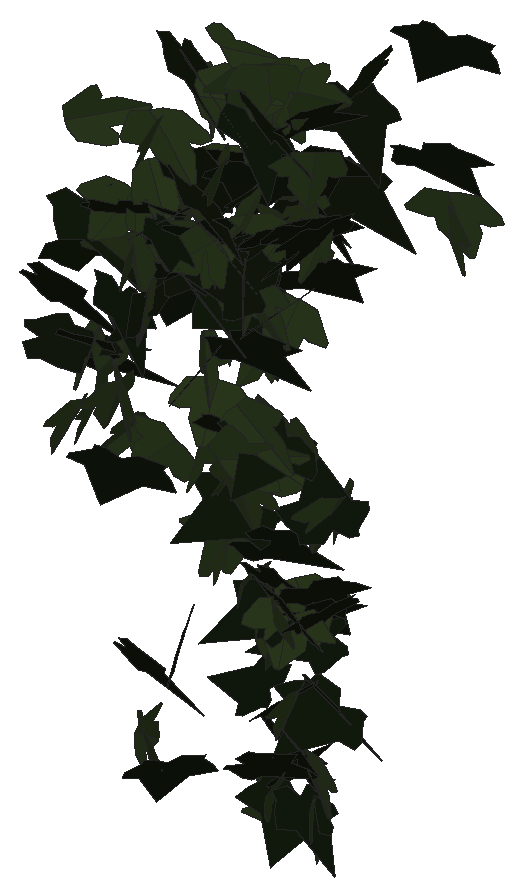
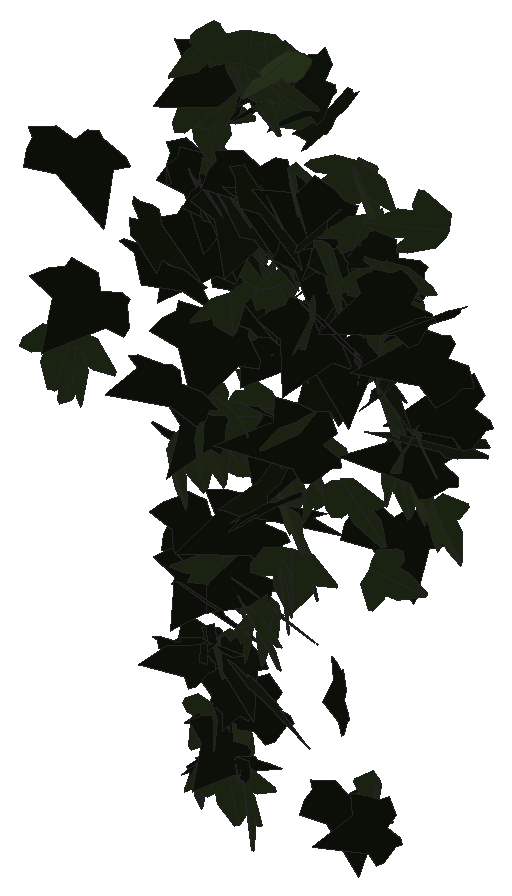
# SketchUp Ruby script. Lengths in inches.
U = 1.inch
M = Sketchup.active_model
def pt(a) = Geom::Point3d.new(a.map { |v| v * U })
def face(e, loops, mat)
  f = e.add_face(loops[0].map { |a| pt(a) })
  loops[1..].each { |l| e.add_face(l.map { |a| pt(a) }).erase! }
  f.material = f.back_material = mat if mat
  f
end
# faces: each face lists its corners as indices into pts; further lists are holes
def faces(e, pts, list, mat = nil) = list.each { |f| face(e, (f[0].is_a?(Array) ? f : [f]).map { |l| l.map { |i| pts[i] } }, mat) }
# xy, xz, yz: faces in a plane at the given z, y or x. An outline is a flat list of corners, or four numbers for a rectangle; further outlines are holes
def ring(l) = l.size == 4 ? [[l[0], l[1]], [l[2], l[1]], [l[2], l[3]], [l[0], l[3]]] : l.each_slice(2).to_a
def flat(e, list, mat, &to3) = list.each { |f| face(e, (f[0].is_a?(Array) ? f : [f]).map { |l| ring(l).map { |u, v| to3.(u, v) } }, mat) }
def xy(e, z, list, mat = nil) = flat(e, list, mat) { |x, y| [x, y, z] }
def xz(e, y, list, mat = nil) = flat(e, list, mat) { |x, z| [x, y, z] }
def yz(e, x, list, mat = nil) = flat(e, list, mat) { |y, z| [x, y, z] }
def lines(e, pts, list) = list.each { |a, b| e.add_line(pt(pts[a]), pt(pts[b])) }
# prism: a flat outline (further loops are holes) pulled along v
def prism(e, loops, v, mat = nil)
  f = face(e, loops, mat); d = Geom::Vector3d.new(v.map { |x| x * U })
  f.pushpull(f.normal.samedirection?(d) ? d.length : -d.length)
end
def box(e, o, s, mat = nil) = prism(e, [[o, [o[0] + s[0], o[1], o[2]], [o[0] + s[0], o[1] + s[1], o[2]], [o[0], o[1] + s[1], o[2]]]], [0, 0, s[2]], mat)
def at(x, y, z, deg = 0) = Geom::Transformation.translation(pt([x, y, z])) * Geom::Transformation.rotation(ORIGIN, Z_AXIS, deg.degrees)
def axes(o, x, y, z) = Geom::Transformation.new([*x, 0, *y, 0, *z, 0, *pt(o).to_a, 1])
def part(name) = M.definitions.add(name)
# library, detail: a bought-in or finely detailed component or shape, given as its bounding box
def library(name, o, s) = part(name).tap { |d| box(d.entities, o, s) }
def detail(e, o, s) = box(e.add_group.entities, o, s)
def put(e, d, t, mat = nil) = e.add_instance(d, t).tap { |i| i.material = mat if mat }
def group(e, t, mat = nil) = e.add_group.tap { |g| g.transformation = t; g.material = mat if mat }.entities
root = M.entities
M.materials.add("1026 AP 7946 SUNNY SIDE UP").color = [254, 231, 186]
M.materials.add("efeu1").color = [18, 25, 13]
M.materials.add("efeu2").color = [43, 57, 29]
c1 = part("ivyleaf_9")
p = [[1.54,2.16,1.25],[1.36,2.04,1.19],[-0.21,0.99,0.68],[-0.71,1.11,0.82],[-0.85,0.86,0.67],[-0.8,0.17,0.21],
  [-0.9,-0.01,0.1],[-0.67,-0.16,-0.02],[-0.08,-0.08,-0.05],[-0.03,-0.6,-0.4],[0.65,-0.88,-0.66],[0.83,-0.6,-0.49],
  [1.29,-0.42,-0.43],[1.8125,-0.07,-0.26],[1.21,0.44,0.15]]
faces(c1.entities,p,[[0,1,2,3,4,5,6,7,8,9,10,11,12,13,14]],"efeu1")
c2 = part("ivyleaf_10")
p = [[0,0.5,-0.03],[-0.0625,2.02,-0.43],[-0.19,2.01,-0.46],[-0.54,1.05,-0.29],[-0.52,0.625,-0.18],[-0.83,0.76,-0.28],
  [-1.16,0.64,-0.33],[-1.15,0.33,-0.24],[-0.77,-0.39,0.02],[-0.3,-0.51,0.16],[0.04,-0.48,0.23],[-0.02,2.01,-0.4375],
  [-0.06,2.01,-0.43],[0.04,-0.49,0.23],[0.67,-0.49,0.14],[1.38,0.36,-0.2],[1.375,0.51,-0.24],[0.81,0.65,-0.19],
  [0.62,0.59,-0.15],[0.6,1.09,-0.28],[0.5,1.23,-0.31]]
faces(c2.entities,p,[[0,1,2,3,4,5,6,7,8,9,10],[11,12,0,13,14,15,16,17,18,19,20]],"efeu2")
put(root,c1,axes([142.16,212.56,287.88],[0.31672,-0.17913,-0.21468],[-0.14461,0.19825,-0.26729],[0.40589,0.21041,0.07229]),"1026 AP 7946 SUNNY SIDE UP")
put(root,c1,axes([143.47,212.86,289.68],[-0.00222,-0.34743,0.04563],[0.00185,-0.04627,-0.35819],[0.55112,-0.00124,0.00138]),"1026 AP 7946 SUNNY SIDE UP")
put(root,c2,axes([140.59,212.77,284.56],[0.03264,-0.32635,0.0778],[0.00053,-0.0775,-0.33731],[0.52738,0.02028,-0.00447]),"1026 AP 7946 SUNNY SIDE UP")
put(root,c1,axes([142.63,212.65,290.1875],[0.46687,-0.18789,-0.08433],[-0.13261,0.01726,-0.36058],[0.29298,0.30723,-0.02883]),"1026 AP 7946 SUNNY SIDE UP")
put(root,c2,axes([140.9375,212.78,284.84],[0.14419,-0.31737,0.06756],[0.0106,-0.06814,-0.3405],[0.51005,0.09114,-0.01202]),"1026 AP 7946 SUNNY SIDE UP")
put(root,c1,axes([143.65,212.61,287.42],[-0.33217,0.19685,0.19333],[-0.25259,0.09968,-0.2952],[-0.34358,-0.26361,0.03012]),"1026 AP 7946 SUNNY SIDE UP")
put(root,c2,axes([141.86,212.79,289.05],[0.19034,-0.32252,0.0712],[0.02553,-0.06966,-0.35518],[0.51864,0.12179,-0.00865]),"1026 AP 7946 SUNNY SIDE UP")
put(root,c2,axes([142.76,212.67,287.71],[0.4264,-0.09253,-0.1913],[-0.25983,0.08705,-0.2936],[0.19605,0.31662,0.02696]),"1026 AP 7946 SUNNY SIDE UP")
put(root,c2,axes([142.76,212.76,286.2],[-0.05936,0.31516,-0.1308],[-0.00302,-0.12974,-0.32734],[-0.53531,-0.03421,0.01635]),"1026 AP 7946 SUNNY SIDE UP")
put(root,c1,axes([140.3,212.55,285.57],[0.47791,-0.13836,-0.01708],[0.18522,0.27565,-0.15089],[0.11681,0.12901,0.30914]),"1026 AP 7946 SUNNY SIDE UP")
put(root,c1,axes([143.61,212.52,280.59],[0.36711,0.09399,0.18355],[0.23946,0.09493,-0.25739],[-0.2062,0.27758,0.02787]),"1026 AP 7946 SUNNY SIDE UP")
put(root,c1,axes([143.52,212.68,290.04],[0.42455,-0.20723,-0.10023],[-0.11046,0.06627,-0.35011],[0.34178,0.27883,0.01135]),"1026 AP 7946 SUNNY SIDE UP")
put(root,c2,axes([141.41,212.75,287.85],[0.50222,-0.0578,-0.10915],[-0.16664,0.00717,-0.33414],[0.08986,0.33633,-0.00961]),"1026 AP 7946 SUNNY SIDE UP")
put(root,c1,axes([141.44,212.66,284.14],[0.28343,0.19809,-0.21343],[-0.21625,-0.15647,-0.27681],[-0.3969,0.22671,-0.00159]),"1026 AP 7946 SUNNY SIDE UP")
put(root,c2,axes([140.83,212.85,285.63],[0.26202,-0.27117,0.11252],[0.07438,-0.10084,-0.32825],[0.45454,0.17282,-0.01114]),"1026 AP 7946 SUNNY SIDE UP")
put(root,c1,axes([143.88,212.92,282.7],[0.41796,-0.19174,-0.06549],[0.10057,-0.01789,0.33674],[-0.30073,-0.27247,0.02159]),"1026 AP 7946 SUNNY SIDE UP")
put(root,c2,axes([141.97,212.79,289.13],[-0.48106,-0.08245,-0.15722],[0.26993,-0.1057,-0.29724],[0.03426,-0.32492,0.13437]),"1026 AP 7946 SUNNY SIDE UP")
put(root,c2,axes([141.27,212.76,285.1],[-0.08842,-0.33307,-0.01997],[-0.00628,0.01841,-0.3478],[0.5244,-0.05594,-0.00753]),"1026 AP 7946 SUNNY SIDE UP")
put(root,c1,axes([141.53,212.54,287.91],[0.46791,0.17457,0.03296],[-0.00239,0.06308,-0.35051],[-0.27879,0.29246,0.05833]),"1026 AP 7946 SUNNY SIDE UP")
put(root,c1,axes([142.49,212.87,287.89],[0.32234,-0.2378,0.14496],[0.12261,-0.12005,-0.32364],[0.41795,0.21862,-0.01686]),"1026 AP 7946 SUNNY SIDE UP")
put(root,c2,axes([141.93,212.72,288.41],[0.15342,0.33367,0.00693],[0.02503,0.00037,-0.35779],[-0.52412,0.09769,-0.01506]),"1026 AP 7946 SUNNY SIDE UP")
put(root,c1,axes([141.25,212.93,286.34],[0.08292,-0.32503,0.06933],[0.00911,-0.0691,-0.33958],[0.52243,0.05279,-0.00508]),"1026 AP 7946 SUNNY SIDE UP")
put(root,c2,axes([143.42,212.79,290.33],[-0.2273,-0.32529,-0.00116],[0.03301,-0.01012,-0.36599],[0.51043,-0.1442,0.02316]),"1026 AP 7946 SUNNY SIDE UP")
put(root,c1,axes([140.13,212.73,286.28],[0.50384,-0.06943,0.10649],[0.14944,-0.0497,-0.33689],[0.1273,0.33312,-0.02599]),"1026 AP 7946 SUNNY SIDE UP")
put(root,c2,axes([141.75,212.91,286.57],[-0.15587,0.24483,-0.21465],[-0.05442,-0.22625,-0.25654],[-0.504,-0.05129,0.09409]),"1026 AP 7946 SUNNY SIDE UP")
put(root,c1,axes([142.63,212.49,285.71],[0.10212,0.17352,0.29558],[0.11716,0.27644,-0.18865],[-0.51269,0.09773,0.01577]),"1026 AP 7946 SUNNY SIDE UP")
put(root,c1,axes([142.32,212.91,286.91],[0.30518,-0.23665,0.14942],[0.11142,-0.13056,-0.31499],[0.42312,0.20507,-0.02483]),"1026 AP 7946 SUNNY SIDE UP")
put(root,c2,axes([143.7,212.8,290.42],[-0.39098,-0.25354,-0.02248],[0.08714,-0.02619,-0.36111],[0.39034,-0.24811,0.0581]),"1026 AP 7946 SUNNY SIDE UP")
put(root,c2,axes([143.3,212.9,287.36],[-0.07804,0.28364,-0.19907],[-0.00288,-0.19707,-0.29623],[-0.54109,-0.03986,0.03029]),"1026 AP 7946 SUNNY SIDE UP")
put(root,c2,axes([142.8125,212.84,289.79],[0.1731,-0.10102,-0.34571],[0.51755,-0.08925,0.13863],[-0.18666,-0.34114,0.06379]),"1026 AP 7946 SUNNY SIDE UP")
put(root,c2,axes([141.36,212.77,285.12],[-0.29905,0.27961,-0.00111],[-0.0498,-0.02474,-0.34606],[-0.43685,-0.18859,0.04021]),"1026 AP 7946 SUNNY SIDE UP")
put(root,c2,axes([143.27,212.71,284.76],[-0.23022,-0.06113,0.32123],[0.40967,0.17411,0.16203],[-0.28695,0.29761,-0.0264]),"1026 AP 7946 SUNNY SIDE UP")
put(root,c1,axes([144.53,212.75,288.5],[-0.02244,0.32187,-0.1215],[0.01837,-0.11935,-0.33255],[-0.5397,-0.01744,-0.00627]),"1026 AP 7946 SUNNY SIDE UP")
put(root,c2,axes([142.89,212.8,283.4],[0.2833,-0.26988,-0.12793],[-0.0952,0.107,-0.33355],[0.4563,0.18988,0.00984]),"1026 AP 7946 SUNNY SIDE UP")
put(root,c1,axes([143.96,212.75,287.16],[-0.13834,0.32899,-0.06288],[-0.00004,-0.06504,-0.3508],[-0.52667,-0.08641,0.01654]),"1026 AP 7946 SUNNY SIDE UP")
put(root,c2,axes([143.26,212.89,285.27],[0.29449,0.02872,0.30171],[0.46243,-0.01457,-0.19247],[-0.00496,0.34719,-0.03099]),"1026 AP 7946 SUNNY SIDE UP")
put(root,c2,axes([141.46,212.83,287.22],[-0.49537,-0.13066,-0.03779],[0.06919,-0.0126,-0.35021],[0.20154,-0.31683,0.02734]),"1026 AP 7946 SUNNY SIDE UP")
put(root,c1,axes([143.78,213.02,285.14],[-0.47996,-0.14286,-0.02762],[0.06539,-0.02802,-0.34453],[0.21876,-0.30506,0.04239]),"1026 AP 7946 SUNNY SIDE UP")
put(root,c1,axes([140.6875,212.89,287.49],[0.09591,-0.31038,-0.13725],[0.06514,0.13949,-0.31865],[0.52599,0.03932,0.06449]),"1026 AP 7946 SUNNY SIDE UP")
put(root,c2,axes([141.41,212.88,286],[0.33443,-0.25888,-0.03833],[-0.01811,0.03674,-0.34463],[0.41052,0.21251,0.01602]),"1026 AP 7946 SUNNY SIDE UP")
put(root,c2,axes([142.91,212.86,287.45],[0.11645,0.33223,-0.04196],[0.0038,-0.04417,-0.35071],[-0.52667,0.07314,-0.01181]),"1026 AP 7946 SUNNY SIDE UP")
put(root,c1,axes([142.34,212.96,288.37],[0.25835,-0.3011,0.00141],[0.01395,0.00133,-0.35326],[0.47328,0.16432,0.00964]),"1026 AP 7946 SUNNY SIDE UP")
put(root,c1,axes([141.76,212.68,286.3125],[-0.14678,0.27555,0.1762],[-0.12716,0.15091,-0.29779],[-0.49252,-0.12108,0.02437]),"1026 AP 7946 SUNNY SIDE UP")
put(root,c1,axes([142.52,212.74,287.83],[0.23809,0.30708,-0.0686],[-0.0292,-0.06698,-0.35287],[-0.49381,0.15202,-0.01221]),"1026 AP 7946 SUNNY SIDE UP")
put(root,c2,axes([143.98,212.94,281.49],[0.04182,-0.31057,0.02656],[-0.0045,-0.02789,-0.32124],[0.49024,0.02624,-0.00522]),"1026 AP 7946 SUNNY SIDE UP")
put(root,c1,axes([143.23,212.74,286.45],[0.49329,0.12947,0.06041],[0.10357,-0.00853,-0.34807],[-0.19751,0.3189,-0.03166]),"1026 AP 7946 SUNNY SIDE UP")
put(root,c2,axes([144.32,212.93,289.34],[-0.30427,-0.2864,0.01904],[0.02361,-0.03431,-0.35479],[0.45082,-0.1915,0.03143]),"1026 AP 7946 SUNNY SIDE UP")
put(root,c2,axes([143.18,212.87,284.41],[-0.50747,0.11474,-0.03236],[0.03509,-0.03271,-0.35224],[-0.18401,-0.32267,0.02206]),"1026 AP 7946 SUNNY SIDE UP")
put(root,c1,axes([144.17,212.81,288.06],[-0.1803,0.32466,-0.02629],[0.0001,-0.02899,-0.35474],[-0.5123,-0.11426,0.00918]),"1026 AP 7946 SUNNY SIDE UP")
put(root,c2,axes([142.01,212.91,284.45],[-0.40481,0.05563,0.20355],[-0.32229,-0.06949,-0.25578],[-0.00039,-0.3168,0.08985]),"1026 AP 7946 SUNNY SIDE UP")
put(root,c2,axes([143.84,212.81,282.75],[-0.32257,0.19704,0.14791],[-0.20382,0.06905,-0.29031],[-0.32346,-0.24002,0.03543]),"1026 AP 7946 SUNNY SIDE UP")
put(root,c2,axes([143.87,212.96,282.64],[0.48794,0.11976,-0.01903],[-0.01037,-0.03587,-0.34138],[-0.19041,0.30883,-0.03017]),"1026 AP 7946 SUNNY SIDE UP")
put(root,c2,axes([141.1,212.66,285.4],[0.05447,-0.03817,-0.34463],[0.03874,0.33547,-0.03487],[0.52767,-0.02069,0.03814]),"1026 AP 7946 SUNNY SIDE UP")
put(root,c1,axes([142.13,212.75,287.84],[0.00933,0.34046,0.02747],[-0.03555,0.02508,-0.34984],[-0.53557,0.00427,0.0237]),"1026 AP 7946 SUNNY SIDE UP")
put(root,c1,axes([142.06,212.83,279.91],[0.15068,0.28452,-0.10779],[-0.04153,-0.10318,-0.3098],[-0.47575,0.09912,-0.0071]),"1026 AP 7946 SUNNY SIDE UP")
put(root,c1,axes([140.55,212.85,285.39],[0.41804,-0.04727,0.20609],[0.31859,0.00262,-0.27638],[0.05685,0.33287,0.03342]),"1026 AP 7946 SUNNY SIDE UP")
put(root,c2,axes([143.3,213,287.13],[-0.37555,0.12158,-0.23349],[0.26951,-0.1566,-0.27271],[-0.30281,-0.29017,0.04686]),"1026 AP 7946 SUNNY SIDE UP")
put(root,c1,axes([143.16,213.13,283.9],[-0.45827,-0.11735,0.10801],[-0.12119,-0.08752,-0.32011],[0.21653,-0.29735,0.04943]),"1026 AP 7946 SUNNY SIDE UP")
put(root,c2,axes([143.29,212.97,288.44],[0.2721,-0.30817,-0.0358],[-0.05649,0.01759,-0.36325],[0.48405,0.17528,-0.02227]),"1026 AP 7946 SUNNY SIDE UP")
put(root,c1,axes([143.89,213.1,279.92],[-0.30957,-0.23132,-0.02436],[0.05417,-0.0001,-0.31176],[0.36138,-0.19814,0.02586]),"1026 AP 7946 SUNNY SIDE UP")
put(root,c2,axes([142.82,212.96,288.76],[0.14333,-0.33091,-0.02765],[0.00014,0.02591,-0.35338],[0.52181,0.09089,0.00769]),"1026 AP 7946 SUNNY SIDE UP")
put(root,c1,axes([144.53,212.82,282.97],[0.00246,0.32354,-0.04458],[-0.00128,-0.0451,-0.33358],[-0.51366,0.00166,0.00062]),"1026 AP 7946 SUNNY SIDE UP")
put(root,c1,axes([143.87,212.87,280.95],[0.41611,-0.0656,-0.154],[-0.23226,0.02331,-0.2805],[0.10801,0.30286,-0.0099]),"1026 AP 7946 SUNNY SIDE UP")
put(root,c1,axes([144.52,213.14,281.46],[-0.46048,-0.12389,0.02926],[-0.02478,-0.03715,-0.32653],[0.19857,-0.29194,0.02709]),"1026 AP 7946 SUNNY SIDE UP")
put(root,c1,axes([143.96,212.85,281.51],[-0.0356,0.31177,-0.02183],[-0.00701,-0.02334,-0.3221],[-0.49151,-0.02225,0.00617]),"1026 AP 7946 SUNNY SIDE UP")
put(root,c2,axes([144.52,213.05,284.375],[-0.12679,-0.30587,0.07598],[-0.00355,-0.07736,-0.32585],[0.49537,-0.07884,0.01711]),"1026 AP 7946 SUNNY SIDE UP")
put(root,c2,axes([141.64,212.95,287.83],[0.13179,0.33065,0.00038],[0.0033,-0.00208,-0.35141],[-0.51991,0.0838,-0.00214]),"1026 AP 7946 SUNNY SIDE UP")
put(root,c2,axes([143.79,212.76,280.08],[0.06986,0.1045,0.29352],[-0.24176,0.25538,-0.07045],[-0.4104,-0.13265,0.09147]),"1026 AP 7946 SUNNY SIDE UP")
put(root,c2,axes([144.32,213.07,288.27],[0.37238,-0.24402,0.04444],[0.01846,-0.05047,-0.34954],[0.3896,0.23562,-0.02592]),"1026 AP 7946 SUNNY SIDE UP")
put(root,c2,axes([143.74,213.08,288.04],[-0.43412,-0.13558,0.15373],[-0.13912,-0.14726,-0.30576],[0.28587,-0.27756,0.08466]),"1026 AP 7946 SUNNY SIDE UP")
put(root,c2,axes([141.42,212.88,287.07],[0.13039,-0.27321,-0.19446],[0.02435,0.19597,-0.28643],[0.52021,0.05931,0.06215]),"1026 AP 7946 SUNNY SIDE UP")
put(root,c1,axes([143.59,213.08,282.59],[-0.49432,0.0874,-0.01384],[0.00009,-0.0512,-0.33259],[-0.13916,-0.31049,0.04894]),"1026 AP 7946 SUNNY SIDE UP")
put(root,c1,axes([142.07,213.13,290.06],[0.21639,-0.32629,0.03573],[0.00666,-0.03785,-0.36487],[0.51622,0.13726,-0.01027]),"1026 AP 7946 SUNNY SIDE UP")
put(root,c2,axes([142.39,213.16,284.57],[-0.08855,0.23991,-0.23232],[-0.06393,-0.23344,-0.24527],[-0.51525,-0.01227,0.07036]),"1026 AP 7946 SUNNY SIDE UP")
put(root,c1,axes([144.02,213.07,279.98],[0.08352,-0.28332,-0.10553],[-0.02818,0.09923,-0.29637],[0.47202,0.05605,0.00098]),"1026 AP 7946 SUNNY SIDE UP")
put(root,c2,axes([143.61,213.02,290.09],[0.43594,-0.17603,-0.14875],[-0.20049,0.06654,-0.33774],[0.29539,0.30495,-0.00971]),"1026 AP 7946 SUNNY SIDE UP")
put(root,c1,axes([144.34,212.84,283.23],[0.29985,0.25674,0.02389],[0.03874,0.00874,-0.32908],[-0.40328,0.19173,-0.01385]),"1026 AP 7946 SUNNY SIDE UP")
put(root,c1,axes([144.21,212.87,288.38],[0.22867,0.31016,-0.03807],[-0.00131,-0.04232,-0.35271],[-0.49148,0.14442,-0.01677]),"1026 AP 7946 SUNNY SIDE UP")
put(root,c2,axes([140.74,212.8,288.77],[-0.04769,-0.06745,0.35237],[0.17252,0.32444,0.07774],[-0.52095,0.11362,-0.00651]),"1026 AP 7946 SUNNY SIDE UP")
put(root,c2,axes([141.6,212.95,280.14],[-0.29855,0.23324,0.09884],[-0.10757,0.06624,-0.30925],[-0.38088,-0.20153,0.00986]),"1026 AP 7946 SUNNY SIDE UP")
put(root,c1,axes([144.625,212.91,284.21],[-0.49748,0.0619,-0.04099],[-0.0521,0.03869,0.33077],[0.10364,0.31656,-0.03046]),"1026 AP 7946 SUNNY SIDE UP")
put(root,c1,axes([142.32,212.95,288.33],[0.1492,0.02595,0.33903],[0.51885,-0.00742,-0.09749],[-0.00007,0.34228,-0.02581]),"1026 AP 7946 SUNNY SIDE UP")
put(root,c2,axes([143.83,213.09,279.71],[-0.37195,-0.18294,0.05192],[-0.04196,-0.04934,-0.30749],[0.29586,-0.237,0.02166]),"1026 AP 7946 SUNNY SIDE UP")
put(root,c2,axes([144.25,212.87,290.35],[-0.04716,-0.18337,-0.31095],[0.22339,0.26995,-0.18255],[0.50689,-0.13603,0.05152]),"1026 AP 7946 SUNNY SIDE UP")
put(root,c2,axes([141.64,212.85,280.17],[-0.00162,0.16166,0.28627],[-0.197,0.25475,-0.15217],[-0.46418,-0.10868,0.06358]),"1026 AP 7946 SUNNY SIDE UP")
put(root,c1,axes([143.83,212.92,288.18],[0.15553,0.32687,-0.03929],[-0.01299,-0.03928,-0.35203],[-0.51764,0.0992,-0.00297]),"1026 AP 7946 SUNNY SIDE UP")
put(root,c1,axes([142.14,212.84,281.33],[0.02555,0.02961,0.32533],[0.11595,0.30702,-0.03178],[-0.4848,0.07499,0.00954]),"1026 AP 7946 SUNNY SIDE UP")
put(root,c1,axes([143.66,213.02,288.14],[-0.3052,0.29238,-0.02024],[-0.00536,-0.0278,-0.36121],[-0.46092,-0.19328,0.0176]),"1026 AP 7946 SUNNY SIDE UP")
put(root,c1,axes([140.48,212.83,286.9375],[0.04977,0.1408,-0.31889],[0.06681,0.30761,0.15004],[0.53167,-0.05183,0.011]),"1026 AP 7946 SUNNY SIDE UP")
put(root,c2,axes([143.73,213.17,284.51],[0.22498,0.17238,0.25724],[-0.28753,-0.16996,0.22873],[0.37914,-0.23118,0.02081]),"1026 AP 7946 SUNNY SIDE UP")
put(root,c1,axes([143.36,213.03,288.8],[0.27648,0.24749,-0.18855],[-0.14818,-0.15908,-0.3134],[-0.46215,0.19906,-0.01231]),"1026 AP 7946 SUNNY SIDE UP")
put(root,c1,axes([144.08,212.83,289.85],[0.29732,0.17812,0.2367],[0.21146,0.18806,-0.26427],[-0.40387,0.2296,0.03589]),"1026 AP 7946 SUNNY SIDE UP")
put(root,c1,axes([141.01,212.93,287.6],[0.40147,0.14605,0.17253],[0.25926,0.04462,-0.30028],[-0.23276,0.30161,-0.0369]),"1026 AP 7946 SUNNY SIDE UP")
put(root,c2,axes([144.16,213.14,280.52],[-0.33902,0.2114,-0.09193],[0.06702,-0.08508,-0.31007],[-0.35527,-0.21778,0.02923]),"1026 AP 7946 SUNNY SIDE UP")
put(root,c2,axes([143.9,213.15,287.98],[-0.51905,0.03629,0.10133],[0.15865,0.02422,0.34049],[0.04364,0.34353,-0.03267]),"1026 AP 7946 SUNNY SIDE UP")
put(root,c1,axes([143.66,212.92,288.1],[0.20073,0.31068,0.077],[0.01498,0.07486,-0.34502],[-0.50158,0.12657,0.02051]),"1026 AP 7946 SUNNY SIDE UP")
put(root,c1,axes([143.35,213.04,288.62],[-0.18202,0.33496,-0.02119],[-0.00411,-0.02467,-0.36508],[-0.52786,-0.11531,0.01015]),"1026 AP 7946 SUNNY SIDE UP")
put(root,c1,axes([143.39,212.96,283.53],[0.4127,0.13191,0.16083],[0.22584,0.06001,-0.3021],[-0.22737,0.29904,-0.00816]),"1026 AP 7946 SUNNY SIDE UP")
put(root,c2,axes([142.97,212.94,290.48],[0.41501,-0.16174,-0.17775],[0.20574,0.31473,-0.09642],[0.3085,0.00768,0.30342]),"1026 AP 7946 SUNNY SIDE UP")
put(root,c1,axes([142.22,213.27,287.125],[-0.50538,0.0763,-0.09075],[0.12659,-0.04323,-0.33977],[-0.13321,-0.33056,0.02142]),"1026 AP 7946 SUNNY SIDE UP")
put(root,c2,axes([144.18,213.17,279.79],[-0.07777,0.30811,-0.01072],[-0.08256,-0.02055,-0.31655],[-0.47777,-0.0466,0.05645]),"1026 AP 7946 SUNNY SIDE UP")
put(root,c2,axes([143.98,213.1,285],[-0.24883,0.05166,-0.29874],[-0.38289,0.16284,0.16757],[0.26137,0.28772,-0.03892]),"1026 AP 7946 SUNNY SIDE UP")
put(root,c1,axes([142.9375,213.0625,285.01],[0.41448,0.1902,-0.08895],[-0.12354,-0.0404,-0.33484],[-0.30508,0.27476,0.01475]),"1026 AP 7946 SUNNY SIDE UP")
put(root,c1,axes([141.97,213.14,286.76],[0.34107,0.17842,-0.20471],[-0.22025,-0.14348,-0.2896],[-0.35893,0.25759,-0.01682]),"1026 AP 7946 SUNNY SIDE UP")
put(root,c2,axes([142.74,213.26,284.22],[0.13439,-0.31861,0.00218],[-0.01667,-0.0069,-0.33965],[0.50075,0.08528,-0.01189]),"1026 AP 7946 SUNNY SIDE UP")
put(root,c2,axes([142.4375,213.26,285.2],[0.4365,0.17502,-0.05264],[-0.04192,-0.05493,-0.3368],[-0.28405,0.27706,-0.03119]),"1026 AP 7946 SUNNY SIDE UP")
put(root,c1,axes([144.11,213.25,281.51],[0.3939,-0.17142,0.07182],[0.07272,-0.05729,-0.31233],[0.28235,0.25391,-0.01974]),"1026 AP 7946 SUNNY SIDE UP")
put(root,c2,axes([142.68,213.24,283.35],[-0.49667,-0.06837,0.0236],[-0.02368,-0.03988,-0.33114],[0.11108,-0.31421,0.03494]),"1026 AP 7946 SUNNY SIDE UP")
put(root,c1,axes([144.31,213.28,282.34],[-0.4582,0.11656,0.07075],[-0.12098,-0.01053,-0.32107],[-0.17433,-0.29905,0.03686]),"1026 AP 7946 SUNNY SIDE UP")
put(root,c1,axes([143.34,213.19,282.91],[0.50787,-0.04806,-0.01016],[-0.02171,-0.0279,-0.33518],[0.07394,0.32193,-0.02863]),"1026 AP 7946 SUNNY SIDE UP")
put(root,c2,axes([143.5,213,282.04],[-0.00737,0.11643,-0.31897],[0.00932,0.31029,0.12167],[0.52102,-0.00391,-0.00669]),"1026 AP 7946 SUNNY SIDE UP")
put(root,c2,axes([143.91,213.2,282.875],[0.25447,0.27449,0.07918],[0.07012,0.0611,-0.32782],[-0.44203,0.16771,-0.00642]),"1026 AP 7946 SUNNY SIDE UP")
put(root,c2,axes([142.08,213.24,288.05],[-0.37078,0.22848,0.11392],[-0.23438,-0.00447,-0.32173],[-0.32198,-0.25986,0.10301]),"1026 AP 7946 SUNNY SIDE UP")
put(root,c1,axes([143.37,213.18,281.32],[-0.2552,0.24578,0.12777],[-0.1466,0.08468,-0.30148],[-0.40625,-0.18496,0.02853]),"1026 AP 7946 SUNNY SIDE UP")
put(root,c1,axes([144.07,213.1,282.69],[0.30303,0.25448,0.06843],[0.06659,0.04943,-0.32854],[-0.40757,0.19728,-0.0028]),"1026 AP 7946 SUNNY SIDE UP")
put(root,c1,axes([144.1,213.17,287.57],[0.35638,0.2494,0.061],[0.08225,0.03044,-0.3465],[-0.39406,0.23191,-0.01716]),"1026 AP 7946 SUNNY SIDE UP")
put(root,c1,axes([143.76,213.125,280.27],[0.14355,0.24638,0.1893],[0.1267,0.16428,-0.26927],[-0.46502,0.12082,-0.01493]),"1026 AP 7946 SUNNY SIDE UP")
put(root,c2,axes([144.42,213.46,284.33],[0.15633,-0.30572,0.04094],[0.04897,-0.03341,-0.3308],[0.48264,0.10242,0.0203]),"1026 AP 7946 SUNNY SIDE UP")
put(root,c2,axes([143.27,213.37,279.71],[0.27209,-0.24051,-0.08817],[0.00265,0.10288,-0.2985],[0.40068,0.16264,0.06185]),"1026 AP 7946 SUNNY SIDE UP")
put(root,c1,axes([142.24,213.23,286.96],[0.2793,0.28917,0.04282],[0.06131,0.02281,-0.3488],[-0.45489,0.18062,-0.02072]),"1026 AP 7946 SUNNY SIDE UP")
put(root,c1,axes([142.6875,213.45,286.6],[-0.12424,-0.25074,-0.22188],[0.1448,0.19446,-0.26868],[0.49765,-0.11918,0.02279]),"1026 AP 7946 SUNNY SIDE UP")
put(root,c2,axes([143.48,213.53,286.63],[0.52975,-0.03917,-0.03551],[-0.05913,-0.02818,-0.348],[0.05655,0.33746,-0.03117]),"1026 AP 7946 SUNNY SIDE UP")
put(root,c2,axes([143.66,213.22,289.76],[0.15709,-0.02014,-0.34746],[0.12489,0.34315,0.00514],[0.51621,-0.07689,0.1045]),"1026 AP 7946 SUNNY SIDE UP")
put(root,c2,axes([140.89,213.66,284],[0.01787,0.21251,-0.26331],[-0.28115,-0.21297,-0.19096],[-0.44234,0.14395,0.11074]),"1026 AP 7946 SUNNY SIDE UP")
put(root,c2,axes([142.94,213.32,282.52],[0.03606,0.20506,0.2557],[-0.21635,0.23005,-0.18221],[-0.45612,-0.09291,0.10665]),"1026 AP 7946 SUNNY SIDE UP")
put(root,c1,axes([140.55,213.98,280.5],[0.44519,-0.10333,0.06225],[0.07995,-0.03832,-0.31015],[0.17091,0.28708,-0.01707]),"1026 AP 7946 SUNNY SIDE UP")
put(root,c2,axes([140.88,215.1,288.39],[-0.1178,0.30699,-0.1313],[0.02001,-0.12969,-0.32582],[-0.52333,-0.07406,0.0171]),"1026 AP 7946 SUNNY SIDE UP")
put(root,c1,axes([142.33,215.21,287.75],[0.40921,0.21079,-0.09985],[-0.09979,-0.07727,-0.34489],[-0.35171,0.26717,-0.01831]),"1026 AP 7946 SUNNY SIDE UP")
put(root,c1,axes([141.3125,215.47,285.81],[0.26467,-0.30299,0.03634],[0.01175,-0.03815,-0.35709],[0.47982,0.16807,-0.0113]),"1026 AP 7946 SUNNY SIDE UP")
put(root,c1,axes([142.91,215.49,288.63],[-0.25976,-0.14443,-0.2823],[0.43967,0.06205,-0.20761],[0.2069,-0.31318,0.08677]),"1026 AP 7946 SUNNY SIDE UP")
put(root,c1,axes([143.25,215.58,289.19],[-0.34357,0.15975,-0.21866],[0.19046,-0.18596,-0.27257],[-0.37305,-0.24207,0.06222]),"1026 AP 7946 SUNNY SIDE UP")
put(root,c2,axes([140.75,215.51,287],[0.18231,0.30179,-0.09262],[-0.06219,-0.08293,-0.33346],[-0.492,0.12231,0.00783]),"1026 AP 7946 SUNNY SIDE UP")
put(root,c2,axes([141.82,215.59,288.57],[0.16985,0.31422,-0.09662],[-0.04608,-0.09099,-0.34282],[-0.51436,0.11191,-0.0012]),"1026 AP 7946 SUNNY SIDE UP")
put(root,c2,axes([140.88,215.62,284.73],[0.23903,-0.30714,0.00268],[0.08321,0.02142,-0.34801],[0.47577,0.15056,0.05953]),"1026 AP 7946 SUNNY SIDE UP")
put(root,c1,axes([140.4375,215.48,286.86],[0.4127,0.02552,0.226],[0.3329,0.06718,-0.26877],[-0.0981,0.33532,0.0387]),"1026 AP 7946 SUNNY SIDE UP")
put(root,c1,axes([144.35,215.59,289.97],[0.27336,0.1845,-0.24478],[-0.25599,-0.1745,-0.26218],[-0.39932,0.23817,0.00051]),"1026 AP 7946 SUNNY SIDE UP")
put(root,c2,axes([142.05,215.72,286.52],[-0.00473,-0.33258,0.05795],[0.01542,-0.05821,-0.34281],[0.53065,-0.00127,0.01048]),"1026 AP 7946 SUNNY SIDE UP")
put(root,c2,axes([141.74,215.73,286.84],[-0.39618,0.11399,-0.22126],[0.25289,-0.15503,-0.27921],[-0.28794,-0.29301,0.05921]),"1026 AP 7946 SUNNY SIDE UP")
put(root,c1,axes([140.97,215.73,285.91],[0.09918,-0.3131,-0.1057],[0.04066,0.10707,-0.32522],[0.51562,0.05178,0.04598]),"1026 AP 7946 SUNNY SIDE UP")
put(root,c1,axes([142.1,215.65,286.77],[0.46836,-0.07547,-0.14611],[-0.2181,0.02815,-0.31633],[0.12629,0.32852,-0.00442]),"1026 AP 7946 SUNNY SIDE UP")
put(root,c1,axes([142.46,215.82,287.18],[-0.04124,-0.10215,-0.33298],[0.4211,0.19158,-0.0838],[0.32533,-0.26092,0.06625]),"1026 AP 7946 SUNNY SIDE UP")
put(root,c2,axes([141.15,215.93,284.27],[0.3875,-0.23265,-0.04946],[-0.08933,0.00752,-0.34741],[0.36227,0.25071,-0.03276]),"1026 AP 7946 SUNNY SIDE UP")
put(root,c1,axes([143.82,215.8,288.05],[0.46486,0.17437,0.00621],[0.01878,-0.01035,-0.35332],[-0.27365,0.2955,-0.0137]),"1026 AP 7946 SUNNY SIDE UP")
put(root,c2,axes([144.11,216.02,287.3125],[-0.52451,-0.10324,-0.06165],[0.11523,-0.03918,-0.35491],[0.1475,-0.33652,0.05806]),"1026 AP 7946 SUNNY SIDE UP")
put(root,c2,axes([143.93,216.09,287.0625],[-0.35645,0.25202,-0.09849],[0.07191,-0.08904,-0.34881],[-0.4185,-0.22995,0.02396]),"1026 AP 7946 SUNNY SIDE UP")
